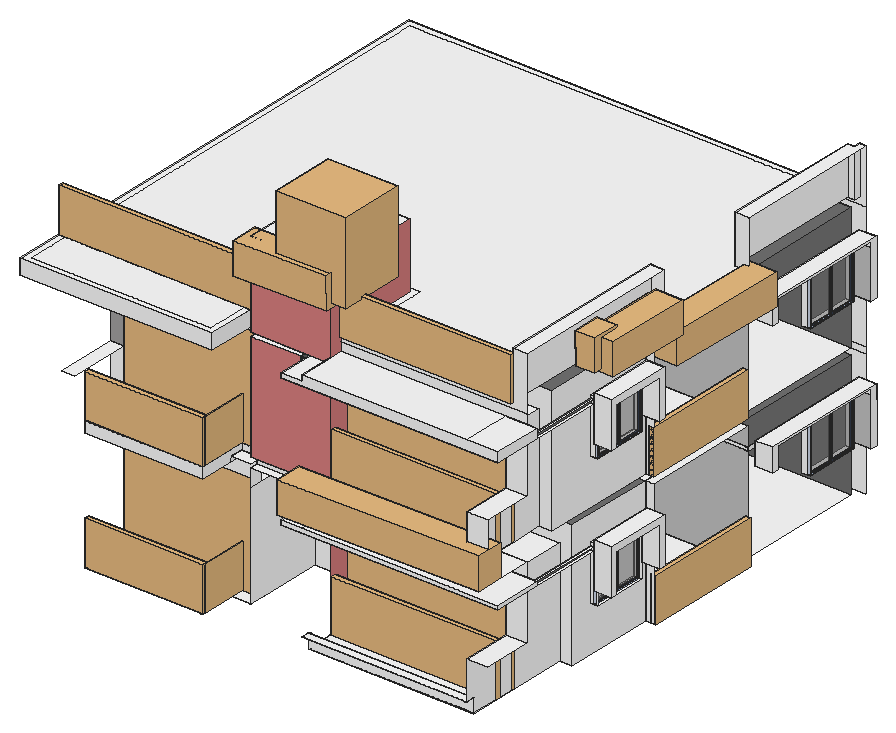
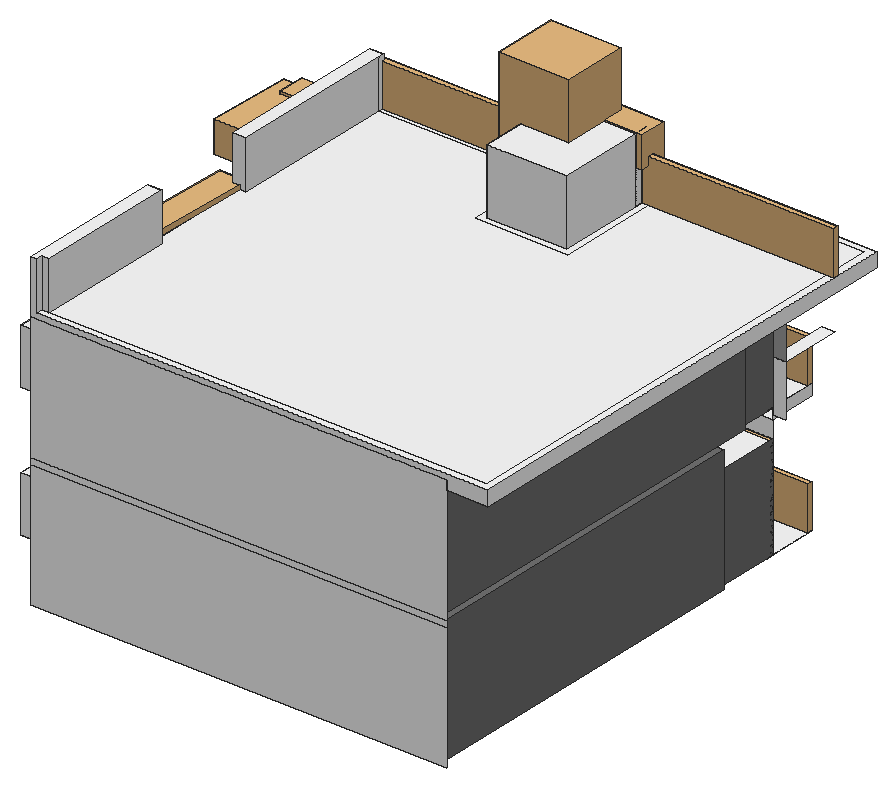
# SketchUp Ruby script. Lengths in inches.
U = 1.inch
M = Sketchup.active_model
def pt(a) = Geom::Point3d.new(a.map { |v| v * U })
def face(e, loops, mat)
  f = e.add_face(loops[0].map { |a| pt(a) })
  loops[1..].each { |l| e.add_face(l.map { |a| pt(a) }).erase! }
  f.material = f.back_material = mat if mat
  f
end
# faces: each face lists its corners as indices into pts; further lists are holes
def faces(e, pts, list, mat = nil) = list.each { |f| face(e, (f[0].is_a?(Array) ? f : [f]).map { |l| l.map { |i| pts[i] } }, mat) }
# xy, xz, yz: faces in a plane at the given z, y or x. An outline is a flat list of corners, or four numbers for a rectangle; further outlines are holes
def ring(l) = l.size == 4 ? [[l[0], l[1]], [l[2], l[1]], [l[2], l[3]], [l[0], l[3]]] : l.each_slice(2).to_a
def flat(e, list, mat, &to3) = list.each { |f| face(e, (f[0].is_a?(Array) ? f : [f]).map { |l| ring(l).map { |u, v| to3.(u, v) } }, mat) }
def xy(e, z, list, mat = nil) = flat(e, list, mat) { |x, y| [x, y, z] }
def xz(e, y, list, mat = nil) = flat(e, list, mat) { |x, z| [x, y, z] }
def yz(e, x, list, mat = nil) = flat(e, list, mat) { |y, z| [x, y, z] }
def lines(e, pts, list) = list.each { |a, b| e.add_line(pt(pts[a]), pt(pts[b])) }
# prism: a flat outline (further loops are holes) pulled along v
def prism(e, loops, v, mat = nil)
  f = face(e, loops, mat); d = Geom::Vector3d.new(v.map { |x| x * U })
  f.pushpull(f.normal.samedirection?(d) ? d.length : -d.length)
end
def box(e, o, s, mat = nil) = prism(e, [[o, [o[0] + s[0], o[1], o[2]], [o[0] + s[0], o[1] + s[1], o[2]], [o[0], o[1] + s[1], o[2]]]], [0, 0, s[2]], mat)
def at(x, y, z, deg = 0) = Geom::Transformation.translation(pt([x, y, z])) * Geom::Transformation.rotation(ORIGIN, Z_AXIS, deg.degrees)
def axes(o, x, y, z) = Geom::Transformation.new([*x, 0, *y, 0, *z, 0, *pt(o).to_a, 1])
def part(name) = M.definitions.add(name)
# library, detail: a bought-in or finely detailed component or shape, given as its bounding box
def library(name, o, s) = part(name).tap { |d| box(d.entities, o, s) }
def detail(e, o, s) = box(e.add_group.entities, o, s)
def put(e, d, t, mat = nil) = e.add_instance(d, t).tap { |i| i.material = mat if mat }
def group(e, t, mat = nil) = e.add_group.tap { |g| g.transformation = t; g.material = mat if mat }.entities
root = M.entities
M.materials.add("[Color M00]").color = [255, 255, 255]
M.materials.add("[Color M02]").color = [198, 198, 198]
M.materials.add("[Color M05]").color = [114, 114, 114]
M.materials.add("[Color M06]").color = [86, 86, 86]
M.materials.add("[Color_006]").color = [86, 86, 86]
M.materials.add("[Stone Vein Gray]").color = [166, 165, 165]
M.materials.add("[Tile Various Tan]").color = [221, 130, 130]
M.materials.add("[Translucent Glass Blue]").color = [74, 111, 178]
M.materials["[Translucent Glass Blue]"].alpha = 0.26
M.materials.add("[Translucent Glass Gray]").color = [128, 128, 128]
M.materials["[Translucent Glass Gray]"].alpha = 0.5
M.materials.add("[Translucent_Glass_Gray]").color = [167, 187, 214]
M.materials["[Translucent_Glass_Gray]"].alpha = 0.8
c1 = library("Glazed balcony doors",[0,0,0],[135.86,2.83,115.35])
c2 = library("Glass Railing",[0,0,0],[139.5,4.76,42])
c3 = part("glass-railing")
detail(c3.entities,[0,0,0],[1.26,75.59,33.1875])
c4 = part("Group\#3")
xy(c4.entities,0,[[0,0,32.48,1.97]])
xy(c4.entities,0.98,[[0.98,0,31.5,0.98],[0.98,0.98,31.5,1.97]])
xy(c4.entities,8.86,[[0.98,0,31.5,0.98],[0.98,0.98,31.5,1.97]])
xy(c4.entities,9.84,[[0,0,32.48,1.97]])
xz(c4.entities,0,[[[0,0,32.48,9.84],[0.98,0.98,31.5,8.86]]])
xz(c4.entities,0.98,[[0.98,0.98,31.5,8.86]],"[Translucent Glass Gray]")
xz(c4.entities,1.97,[[[0,0,32.48,9.84],[0.98,0.98,31.5,8.86]]])
yz(c4.entities,0,[[0,0,1.97,9.84]])
yz(c4.entities,0.98,[[0,0.98,0.98,8.86],[0.98,0.98,1.97,8.86]])
yz(c4.entities,31.5,[[0,0.98,0.98,8.86],[0.98,0.98,1.97,8.86]])
yz(c4.entities,32.48,[[0,0,1.97,9.84]])
c5 = part("Group\#4")
xy(c5.entities,0,[[0,0,32.48,1.97]])
xy(c5.entities,0.98,[[0.98,0,31.5,0.98],[0.98,0.98,31.5,1.97]])
xy(c5.entities,71.85,[[0.98,0,31.5,0.98],[0.98,0.98,31.5,1.97]])
xy(c5.entities,72.83,[[0,0,32.48,1.97]])
xz(c5.entities,0,[[[0,0,32.48,72.83],[0.98,0.98,31.5,71.85]]])
xz(c5.entities,0.98,[[0.98,0.98,31.5,71.85]],"[Translucent Glass Gray]")
xz(c5.entities,1.97,[[[0,0,32.48,72.83],[0.98,0.98,31.5,71.85]]])
yz(c5.entities,0,[[0,0,1.97,72.83]])
yz(c5.entities,0.98,[[0,0.98,0.98,71.85],[0.98,0.98,1.97,71.85]])
yz(c5.entities,31.5,[[0,0.98,0.98,71.85],[0.98,0.98,1.97,71.85]])
yz(c5.entities,32.48,[[0,0,1.97,72.83]])
c6 = part("Fixed transom window")
xy(c6.entities,0,[[0,0,70.86,3.9375]])
xy(c6.entities,1.97,[[1.97,0,34.45,0.98],[36.42,0,68.9,3.9375],[1.97,2.95,34.45,3.9375]])
xy(c6.entities,86.61,[[1.97,0,34.45,3.9375],[34.45,0,36.42,3.9375],[36.42,0,68.9,3.9375]])
xy(c6.entities,88.58,[[0,0,70.86,3.9375]])
xz(c6.entities,0,[[[0,0,70.86,88.58],[1.97,1.97,34.45,86.61],[36.42,1.97,68.9,86.61]]])
xz(c6.entities,3.9375,[[[0,0,70.86,88.58],[1.97,1.97,34.45,86.61],[36.42,1.97,68.9,86.61]]])
yz(c6.entities,0,[[0,0,3.9375,88.58]])
yz(c6.entities,1.97,[[0,1.97,3.9375,74.8],[0,76.77,3.9375,86.61]])
yz(c6.entities,34.45,[[0,1.97,3.9375,86.61]])
yz(c6.entities,36.42,[[0,1.97,3.9375,86.61]])
yz(c6.entities,68.9,[[0,1.97,3.9375,86.61]])
yz(c6.entities,70.86,[[0,0,3.9375,88.58]])
g1 = group(c6.entities,at(1.97,0,74.8))
box(g1,[0,0,0],[66.93,3.9375,1.97])
put(c6.entities,c4,at(1.97,0.98,76.77),"[Translucent Glass Blue]")
put(c6.entities,c4,at(36.42,0.98,76.77),"[Translucent Glass Blue]")
put(c6.entities,c5,at(1.97,0.98,1.97),"[Translucent Glass Blue]")
put(c6.entities,c5,at(36.42,0.98,1.97),"[Translucent Glass Blue]")
c7 = part("FIXED+GLASS+WINDOW+WITH+TRANSOM")
put(c7.entities,c6,at(0,0,0),"[Translucent Glass Blue]")
c8 = part("BIC_Bike Shop - Window - Small")
xy(c8.entities,-8,[[[0,0,36,36],[2,2,34,34]]],"[Color_006]")
xy(c8.entities,-4,[[2,2,34,34]],"[Translucent_Glass_Gray]")
xy(c8.entities,0,[[[0,0,36,36],[2,2,34,34]]],"[Color_006]")
xz(c8.entities,0,[[0,-8,36,0]],"[Color_006]")
xz(c8.entities,2,[[2,-8,34,-4],[2,-4,34,0]],"[Color_006]")
xz(c8.entities,34,[[2,-8,34,-4],[2,-4,34,0]],"[Color_006]")
xz(c8.entities,36,[[0,-8,36,0]],"[Color_006]")
yz(c8.entities,0,[[0,-8,36,0]],"[Color_006]")
yz(c8.entities,2,[[2,-8,34,-4],[2,-4,34,0]],"[Color_006]")
yz(c8.entities,34,[[2,-8,34,-4],[2,-4,34,0]],"[Color_006]")
yz(c8.entities,36,[[0,-8,36,0]],"[Color_006]")
c9 = library("Living wall panel",[-0.54,-4.26,-5.13],[55.52,26.12,125.59])
c10 = library("Flora+17",[-57.52,158.6,-38.64],[66.99,62.88,77.28])
xy(root,635.5625,[[73.74,83.25,73.74,137.58,204.98,137.58,204.98,117.625,186.35,117.625,186.35,83.25],[281.18,91.3,439.11,137.58],[73.74,137.58,204.98,137.58,204.98,194.2,281.18,194.2,281.18,137.58,439.11,137.58,439.11,194.2,450.92,194.2,450.92,281.78,343.48,281.78,343.48,394.46,450.92,394.46,450.92,527.42,69.2,527.42,69.2,194.2,73.74,194.2],[343.48,281.78,450.92,290.48],[450.92,281.78,458.625,394.46],
  [343.48,290.48,352.1875,394.46],[352.1875,290.48,450.92,394.46]],"[Color M00]")
xy(root,635.8125,[[73.74,83.25,186.35,83.25,186.35,117.625,204.98,117.625,204.98,137.58,73.74,137.58],[281.18,91.3,439.11,137.58]],"[Color M00]")
xy(root,649,[[281.18,83.25,439.11,91.3]],"[Color M00]")
xy(root,649.25,[[281.18,83.25,439.11,91.3]],"[Color M00]")
xy(root,679.98,[[450.92,215.57,458.625,267.63],[450.92,468.92,458.625,520.98]],"[Color M00]")
xy(root,685.84,[[439.11,83.25,458.625,129.875]],"[Color M00]")
xy(root,686.24,[[458.625,520.98,475.1875,526.98]],"[Color M00]")
xy(root,694.95,[[458.625,210.07,475.5625,215.57],[458.625,267.63,475.5625,273.63]],"[Color M00]")
xy(root,717.36,[[458.625,402.98,475.1875,408.98]],"[Color M00]")
xy(root,718.41,[[252.64,117.625,281.18,122.0625]],"[Tile Various Tan]")
xy(root,729.27,[[456.375,130.82,458.625,210.07]],"[Color M00]")
xy(root,732.05,[[450.92,215.57,458.625,267.63],[458.625,215.57,475.5625,267.63],[450.92,468.92,458.625,520.98]],"[Color M00]")
xy(root,733.27,[[456.375,130.82,458.625,210.07]],"[Color M00]")
xy(root,734.19,[[381.625,394.46,385.6875,394.83],[385.6875,394.46,401.8125,394.83],[401.8125,394.46,458.625,394.83]],"[Color M00]")
xy(root,734.48,[[73.74,129.875,204.98,194.2]],"[Color M00]")
xy(root,736.125,[[281.18,129.875,439.11,194.2]],"[Color M00]")
xy(root,737.48,[[381.625,394.46,385.6875,394.83],[385.6875,394.46,401.8125,394.83],[401.8125,394.46,458.625,394.83],[458.625,394.46,459,400.46]],"[Color M00]")
xy(root,737.49,[[458.625,408.98,475.1875,520.98]],"[Color M02]")
xy(root,738.39,[[261.54,83.25,261.54,122.0625,281.18,122.0625,281.18,129.875,468.99,129.875,468.99,83.25]],"[Color M00]")
xy(root,738.39,[[252.64,117.625,261.54,122.0625]],"[Tile Various Tan]")
xy(root,738.64,[[458.625,210.07,475.5625,273.63]],"[Color M00]")
xy(root,739.3,[[458.625,402.98,475.1875,526.98]],"[Color M00]")
xy(root,742.08,[[261.54,83.25,281.18,117.625],[281.18,83.25,468.99,129.875]],"[Color M00]")
xy(root,750.9375,[[[73.74,83.25,186.35,129.875],[129.49,93.91,131.04,94.12,132.49,94.72,133.73,95.67,134.68,96.91,135.28,98.36,135.49,99.91,135.28,101.46,134.68,102.91,133.73,104.15,132.49,105.11,131.04,105.71,129.49,105.91,127.93,105.71,126.49,105.11,125.24,104.15,124.29,102.91,123.69,101.46,123.49,99.91,123.69,98.36,124.29,96.91,125.24,95.67,126.49,94.72,127.93,94.12]]],"[Color M00]")
xy(root,752.39,[[204.98,117.625,279.24,125.0625]],"[Color M00]")
xy(root,752.8125,[[129.49,93.91,127.93,94.12,126.49,94.72,125.24,95.67,124.29,96.91,123.69,98.36,123.49,99.91,123.69,101.46,124.29,102.91,125.24,104.15,126.49,105.11,127.93,105.71,129.49,105.91,131.04,105.71,132.49,105.11,133.73,104.15,134.68,102.91,135.28,101.46,135.49,99.91,135.28,98.36,134.68,96.91,133.73,95.67,132.49,94.72,131.04,94.12]],"[Color M06]")
xy(root,755.5625,[[281.18,83.25,458.625,129.875],[186.35,117.625,204.98,129.875],[279.24,117.625,281.18,117.625,281.18,129.875,204.98,129.875,204.98,125.0625,279.24,125.0625],[343.48,281.78,450.92,290.48],[450.92,281.78,450.92,290.48,352.1875,290.48,352.1875,394.46,458.625,394.46,458.625,281.78],
  [343.48,290.48,352.1875,394.46]],"[Color M00]")
xy(root,755.5625,[[69.2,194.2,69.2,527.42,450.92,527.42,450.92,394.46,343.48,394.46,343.48,281.78,450.92,281.78,450.92,194.2]],"[Color M05]")
xy(root,761.5625,[[73.74,83.25,73.74,137.58,204.98,137.58,204.98,129.875,186.35,129.875,186.35,83.25],[281.18,91.3,439.11,137.58],[204.98,117.625,281.18,129.875],[204.98,129.875,281.18,169.45],[73.74,137.58,204.98,137.58,204.98,169.45,281.18,169.45,281.18,137.58,439.11,137.58,439.11,169.45,450.92,169.45,450.92,281.78,343.48,281.78,343.48,394.46,450.92,394.46,450.92,527.42,69.2,527.42,69.2,169.45,73.74,169.45],
  [343.48,281.78,352.1875,290.48],[352.1875,281.78,450.92,290.48],[450.92,281.78,458.625,394.46],[343.48,290.48,352.1875,394.46],[352.1875,290.48,450.92,394.46]],"[Color M00]")
xy(root,761.8125,[[73.74,83.25,186.35,83.25,186.35,129.875,204.98,129.875,204.98,137.58,73.74,137.58],[281.18,91.3,439.11,137.58]],"[Color M00]")
xy(root,775,[[281.18,83.25,439.11,91.3]],"[Color M00]")
xy(root,775.25,[[281.18,83.25,439.11,91.3]],"[Color M00]")
xy(root,805.18,[[61.5,71.125,73.74,129.875]],"[Color M00]")
xy(root,805.98,[[450.92,215.57,458.625,267.63],[450.92,468.92,458.625,520.98]],"[Color M00]")
xy(root,811.84,[[439.11,83.25,458.625,129.875]],"[Color M00]")
xy(root,812.24,[[458.625,520.98,475.1875,526.98]],"[Color M00]")
xy(root,820.95,[[458.625,210.07,475.5625,215.57],[458.625,267.63,475.5625,273.63]],"[Color M00]")
xy(root,843.36,[[458.625,402.98,475.1875,408.98]],"[Color M00]")
xy(root,844.41,[[252.64,117.625,281.18,122.0625]],"[Tile Various Tan]")
xy(root,855.27,[[456.375,130.82,458.625,210.07]],"[Color M00]")
xy(root,858.05,[[450.92,215.57,458.625,267.63],[458.625,215.57,475.5625,267.63],[450.92,468.92,458.625,520.98]],"[Color M00]")
xy(root,859.27,[[456.375,130.82,458.625,210.07]],"[Color M00]")
xy(root,860.19,[[381.625,394.46,385.6875,396.71],[385.6875,394.46,401.8125,396.71],[401.8125,394.46,458.625,396.71]],"[Color M00]")
xy(root,860.48,[[73.74,129.875,204.98,169.45]],"[Color M00]")
xy(root,862.125,[[281.18,129.875,439.11,169.45]],"[Color M00]")
xy(root,863.48,[[381.625,394.46,385.6875,396.71],[385.6875,394.46,401.8125,396.71],[401.8125,394.46,458.625,396.71],[458.625,394.46,459,400.46]],"[Color M00]")
xy(root,863.49,[[458.625,408.98,475.1875,520.98]],"[Color M00]")
xy(root,864.39,[[261.54,83.25,261.54,122.0625,281.18,122.0625,281.18,129.875,468.99,129.875,468.99,83.25],[204.98,117.625,252.64,117.625,252.64,122.0625,261.54,122.0625,261.54,137.1875,204.98,137.1875]],"[Color M00]")
xy(root,864.64,[[458.625,210.07,475.5625,273.63]],"[Color M00]")
xy(root,865.3,[[458.625,402.98,475.1875,526.98]],"[Color M00]")
xy(root,868.08,[[261.54,83.25,281.18,117.625],[204.98,117.625,261.54,137.1875]],"[Color M00]")
xy(root,873.0625,[[[22.125,71.125,22.125,535.125,61.5,535.125,61.5,129.875,204.98,129.875,204.98,71.125],[124.6,84.17,126.16,84.38,127.6,84.98,128.85,85.93,129.8,87.17,130.4,88.62,130.6,90.17,130.4,91.73,129.8,93.17,128.85,94.42,127.6,95.37,126.16,95.97,124.6,96.17,123.05,95.97,121.6,95.37,120.36,94.42,119.41,93.17,118.81,91.73,118.6,90.17,118.81,88.62,119.41,87.17,120.36,85.93,121.6,84.98,123.05,84.38]]],"[Color M00]")
xy(root,873.08,[[281.18,83.25,439.24,129.875],[439.24,83.25,468.99,129.875]],"[Color M00]")
xy(root,874.9375,[[124.6,84.17,123.05,84.38,121.6,84.98,120.36,85.93,119.41,87.17,118.81,88.62,118.6,90.17,118.81,91.73,119.41,93.17,120.36,94.42,121.6,95.37,123.05,95.97,124.6,96.17,126.16,95.97,127.6,95.37,128.85,94.42,129.8,93.17,130.4,91.73,130.6,90.17,130.4,88.62,129.8,87.17,128.85,85.93,127.6,84.98,126.16,84.38]],"[Color M06]")
xy(root,881.5625,[[343.48,281.78,352.1875,290.48],[352.1875,281.78,450.92,290.48],[450.92,281.78,450.92,290.48,352.1875,290.48,352.1875,394.46,458.625,394.46,458.625,281.78],[343.48,290.48,352.1875,394.46]],"[Color M00]")
xy(root,881.5625,[[69.2,169.45,69.2,527.42,450.92,527.42,450.92,394.46,343.48,394.46,343.48,281.78,450.92,281.78,450.92,169.45]],"[Color M05]")
xy(root,887.5625,[[22.125,71.125,204.98,71.125,204.98,212.5625,281.18,212.5625,281.18,129.875,445.9,129.875,445.9,135.91,287.21,135.91,287.21,218.6,198.94,218.6,198.94,77.16,28.16,77.16,28.16,529.09,452.59,529.09,452.59,535.125,22.125,535.125],[28.16,77.16,198.94,77.16,198.94,218.6,287.21,218.6,287.21,135.91,445.9,135.91,445.9,293.73,452.59,293.73,452.59,395.21,445.9,395.21,445.9,529.09,28.16,529.09],[452.59,293.73,458.625,395.21]],"[Color M00]")
xy(root,898.34,[[458.625,209.21,475.5625,275.34]],"[Color M00]")
xy(root,921.66,[[458.625,209.21,475.5625,275.34]],"[Color M00]")
xy(root,933.5,[[445.9,129.875,458.625,293.73],[445.9,395.21,458.625,395.21,458.625,535.125,452.59,535.125,452.59,529.09,445.9,529.09]],"[Color M00]")
xy(root,950.125,[[204.98,117.625,281.18,129.875],[204.98,129.875,281.18,212.5625]],"[Color M00]")
xz(root,71.125,[[22.125,873.0625,204.98,887.5625]],"[Color M00]")
xz(root,83.25,[[73.74,635.5625,186.35,635.8125],[281.18,649,439.11,649.25],[261.54,738.39,468.99,742.08],[73.74,750.9375,186.35,761.5625],[281.18,755.5625,458.625,755.5625,458.625,811.84,439.11,811.84,439.11,775,281.18,775],
  [73.74,761.5625,186.35,761.8125],[281.18,775,439.11,775.25],[261.54,864.39,468.99,864.39,468.99,873.08,281.18,873.08,281.18,868.08,261.54,868.08]],"[Color M00]")
xz(root,91.3,[[281.18,635.5625,439.11,635.8125],[281.18,635.8125,439.11,649],[281.18,649,439.11,649.25],[281.18,761.5625,439.11,761.8125],[281.18,761.8125,439.11,775],
  [281.18,775,439.11,775.25]],"[Color M00]")
xz(root,117.625,[[186.35,635.5625,204.98,635.8125],[279.24,742.08,281.18,755.5625]],"[Color M00]")
xz(root,117.625,[[204.98,761.5625,281.18,761.5625,281.18,844.41,252.64,844.41,252.64,864.39,204.98,864.39],[204.98,868.08,281.18,950.125]],"[Tile Various Tan]")
xz(root,122.0625,[[252.64,718.41,281.18,738.39],[252.64,844.41,281.18,864.39]],"[Tile Various Tan]")
xz(root,125.0625,[[204.98,752.39,279.24,755.5625]],"[Color M00]")
xz(root,129.875,[[439.11,685.84,458.625,685.84,458.625,738.39,281.18,738.39,281.18,736.125,439.11,736.125],[73.74,734.48,204.98,734.48,204.98,755.5625,186.35,755.5625,186.35,750.9375,73.74,750.9375],[439.24,738.39,458.625,742.08],[458.625,738.39,468.99,742.08],[281.18,742.08,458.625,755.5625],
  [61.5,755.5625,73.74,805.18],[186.35,755.5625,281.18,761.5625],[186.35,761.5625,204.98,761.8125],[439.11,811.84,458.625,811.84,458.625,864.39,281.18,864.39,281.18,862.125,439.11,862.125],[73.74,860.48,204.98,873.0625],
  [439.24,864.39,458.625,873.08],[458.625,864.39,468.99,873.08],[61.5,873.0625,204.98,881.5625],[281.18,873.08,458.625,881.5625],[281.18,881.5625,458.625,881.5625,458.625,933.5,445.9,933.5,445.9,887.5625,281.18,887.5625]],"[Color M00]")
xz(root,129.875,[[61.5,805.18,73.74,873.0625]],"[Stone Vein Gray]")
xz(root,130.82,[[456.375,729.27,458.625,733.27],[456.375,855.27,458.625,859.27]],"[Color M00]")
xz(root,137.1875,[[204.98,864.39,261.54,868.08]],"[Color M00]")
xz(root,137.58,[[73.74,635.5625,204.98,635.8125],[281.18,635.5625,439.11,635.8125],[73.74,761.5625,204.98,761.8125],[281.18,761.5625,439.11,761.8125]],"[Color M00]")
xz(root,169.45,[[69.2,761.5625,69.2,881.5625,450.92,881.5625,450.92,761.5625,439.11,761.5625,439.11,862.125,281.18,862.125,281.18,761.5625,204.98,761.5625,204.98,860.48,73.74,860.48,73.74,761.5625]],"[Color M00]")
xz(root,194.2,[[69.2,635.5625,69.2,755.5625,450.92,755.5625,450.92,635.5625,439.11,635.5625,439.11,736.125,281.18,736.125,281.18,635.5625,204.98,635.5625,204.98,734.48,73.74,734.48,73.74,635.5625]],"[Color M00]")
xz(root,209.21,[[458.625,898.34,475.5625,921.66]],"[Color M00]")
xz(root,210.07,[[458.625,694.95,475.5625,738.64],[456.375,729.27,458.625,732.11],[456.375,732.11,458.625,733.27],[458.625,820.95,475.5625,864.64],[456.375,855.27,458.625,858.11],
  [456.375,858.11,458.625,859.27]],"[Color M00]")
xz(root,212.5625,[[204.98,887.5625,281.18,950.125]],"[Color M00]")
xz(root,215.57,[[450.92,679.98,458.625,732.05],[458.625,694.95,475.5625,732.05],[450.92,805.98,458.625,858.05],[458.625,820.95,475.5625,858.05]],"[Color M00]")
xz(root,267.63,[[450.92,679.98,458.625,732.05],[458.625,694.95,475.5625,732.05],[450.92,805.98,458.625,858.05],[458.625,820.95,475.5625,858.05]],"[Color M00]")
xz(root,273.63,[[458.625,694.95,475.5625,738.64],[458.625,820.95,475.5625,864.64]],"[Color M00]")
xz(root,275.34,[[458.625,898.34,475.5625,921.66]],"[Color M00]")
xz(root,281.78,[[343.48,635.5625,450.92,755.5625],[450.92,635.5625,458.625,755.5625],[343.48,761.5625,352.1875,881.5625],[352.1875,761.5625,450.92,881.5625],[450.92,761.5625,458.625,881.5625]],"[Color M00]")
xz(root,290.48,[[343.48,635.5625,352.1875,755.5625],[352.1875,635.5625,450.92,755.5625],[343.48,761.5625,352.1875,881.5625],[352.1875,761.5625,450.92,881.5625]],"[Color M00]")
xz(root,293.73,[[445.9,887.5625,458.625,933.5]],"[Color M00]")
xz(root,394.46,[[343.48,635.5625,352.1875,755.5625],[343.48,761.5625,352.1875,881.5625]],"[Color M00]")
xz(root,394.46,[[352.1875,635.5625,458.625,635.5625,458.625,734.19,381.625,734.19,381.625,737.48,458.625,737.48,458.625,755.5625,352.1875,755.5625],[352.1875,761.5625,458.625,761.5625,458.625,860.19,381.625,860.19,381.625,863.48,458.625,863.48,458.625,881.5625,352.1875,881.5625]],"[Color M02]")
xz(root,394.83,[[381.625,734.19,458.625,737.48]],"[Color M00]")
xz(root,395.21,[[445.9,887.5625,458.625,933.5]],"[Color M00]")
xz(root,396.71,[[381.625,860.19,458.625,863.48]],"[Color M00]")
xz(root,400.46,[[458.625,734.11,459,737.48],[458.625,860.11,459,863.48]],"[Color M00]")
xz(root,402.98,[[458.625,717.36,475.1875,739.3],[458.625,843.36,475.1875,865.3]],"[Color M00]")
xz(root,408.98,[[458.625,717.36,475.1875,731.49],[458.625,731.49,475.1875,737.49],[458.625,843.36,475.1875,857.49],[458.625,857.49,475.1875,863.49]],"[Color M00]")
xz(root,468.92,[[450.92,679.98,458.625,732.05],[450.92,805.98,458.625,858.05]],"[Color M00]")
xz(root,520.98,[[450.92,679.98,458.625,732.05],[458.625,732.05,475.1875,737.49],[450.92,805.98,458.625,858.05],[458.625,858.05,475.1875,863.49]],"[Color M00]")
xz(root,520.98,[[458.625,686.24,475.1875,732.05],[458.625,812.24,475.1875,858.05]],"[Color M02]")
xz(root,526.98,[[458.625,686.24,475.1875,739.3],[458.625,812.24,475.1875,865.3]],"[Color M00]")
xz(root,527.42,[[69.2,635.5625,450.92,755.5625],[69.2,761.5625,450.92,881.5625]],"[Color M05]")
xz(root,529.09,[[445.9,887.5625,452.59,933.5]],"[Color M00]")
xz(root,535.125,[[61.5,635.5625,458.625,755.5625],[61.5,755.5625,458.625,761.5625],[61.5,761.5625,458.625,881.5625],[22.125,873.0625,22.125,887.5625,452.59,887.5625,452.59,933.5,458.625,933.5,458.625,881.5625,61.5,881.5625,61.5,873.0625]],"[Color M00]")
yz(root,22.125,[[71.125,873.0625,535.125,887.5625]],"[Color M00]")
yz(root,61.5,[[129.875,873.0625,535.125,881.5625]],"[Color M00]")
yz(root,69.2,[[194.2,635.5625,527.42,755.5625],[169.45,761.5625,527.42,881.5625]],"[Color M05]")
yz(root,73.74,[[83.25,635.5625,129.875,635.8125],[129.875,635.5625,137.58,635.8125],[83.25,750.9375,129.875,761.5625],[83.25,761.5625,129.875,761.8125],[129.875,761.5625,137.58,761.8125]],"[Color M00]")
yz(root,73.74,[[137.58,635.5625,194.2,635.5625,194.2,734.48,129.875,734.48,129.875,635.8125,137.58,635.8125],[137.58,761.5625,169.45,761.5625,169.45,860.48,129.875,860.48,129.875,761.8125,137.58,761.8125]],"[Color M05]")
yz(root,186.35,[[83.25,635.5625,117.625,635.8125],[83.25,750.9375,117.625,750.9375,117.625,755.5625,129.875,755.5625,129.875,761.5625,83.25,761.5625],[117.625,750.9375,129.875,755.5625],[83.25,761.5625,129.875,761.8125]],"[Color M00]")
yz(root,204.98,[[117.625,635.5625,137.58,635.8125],[137.58,635.5625,137.58,635.8125,117.625,635.8125,117.625,734.48,194.2,734.48,194.2,635.5625],[117.625,734.48,117.625,752.39,125.0625,752.39,125.0625,755.5625,129.875,755.5625,129.875,734.48],[117.625,761.5625,117.625,860.48,169.45,860.48,169.45,761.5625,137.58,761.5625,137.58,761.8125,129.875,761.8125,129.875,761.5625],[129.875,761.5625,137.58,761.8125],
  [117.625,860.48,129.875,864.39],[129.875,864.39,137.1875,868.08],[117.625,868.08,129.875,873.0625],[71.125,873.0625,117.625,887.5625],[117.625,873.0625,129.875,887.5625],
  [117.625,887.5625,129.875,950.125],[129.875,887.5625,212.5625,950.125]],"[Color M00]")
yz(root,252.64,[[117.625,718.41,122.0625,738.39],[117.625,844.41,122.0625,864.39]],"[Tile Various Tan]")
yz(root,261.54,[[83.25,738.39,117.625,742.08],[83.25,864.39,137.1875,868.08]],"[Color M00]")
yz(root,279.24,[[117.625,752.39,125.0625,755.5625]],"[Color M00]")
yz(root,281.18,[[91.3,635.5625,117.625,635.8125],[117.625,635.5625,137.58,635.8125],[83.25,649,91.3,649.25],[122.0625,736.125,129.875,738.39],[117.625,742.08,129.875,755.5625],
  [83.25,755.5625,83.25,775,91.3,775,91.3,761.5625,129.875,761.5625,129.875,755.5625],[91.3,761.5625,117.625,761.8125],[117.625,761.5625,129.875,761.8125],[129.875,761.5625,137.58,761.8125],[83.25,775,91.3,775.25],
  [83.25,868.08,117.625,873.08]],"[Color M00]")
yz(root,281.18,[[137.58,635.5625,194.2,635.5625,194.2,736.125,122.0625,736.125,122.0625,718.41,117.625,718.41,117.625,635.8125,137.58,635.8125],[137.58,761.5625,169.45,761.5625,169.45,862.125,122.0625,862.125,122.0625,844.41,117.625,844.41,117.625,761.8125,137.58,761.8125],[122.0625,862.125,129.875,864.39],[117.625,873.08,129.875,873.08,129.875,887.5625,212.5625,887.5625,212.5625,950.125,117.625,950.125]],"[Tile Various Tan]")
yz(root,343.48,[[281.78,635.5625,290.48,755.5625],[290.48,635.5625,394.46,755.5625],[281.78,761.5625,290.48,881.5625],[290.48,761.5625,394.46,881.5625]],"[Color M00]")
yz(root,352.1875,[[290.48,635.5625,394.46,755.5625],[281.78,761.5625,290.48,881.5625],[290.48,761.5625,394.46,881.5625]],"[Color M00]")
yz(root,381.625,[[394.46,734.19,394.83,737.48],[394.46,860.19,396.71,863.48]],"[Color M00]")
yz(root,439.11,[[137.58,635.5625,137.58,635.8125,91.3,635.8125,91.3,649.25,83.25,649.25,83.25,685.84,129.875,685.84,129.875,736.125,194.2,736.125,194.2,635.5625],[91.3,635.5625,137.58,635.8125],[83.25,649,91.3,649.25],[137.58,761.5625,137.58,761.8125,91.3,761.8125,91.3,775.25,83.25,775.25,83.25,811.84,129.875,811.84,129.875,862.125,169.45,862.125,169.45,761.5625],[91.3,761.5625,137.58,761.8125],
  [83.25,775,91.3,775.25]],"[Color M00]")
yz(root,445.9,[[129.875,887.5625,135.91,933.5],[135.91,887.5625,293.73,933.5],[395.21,887.5625,529.09,933.5]],"[Color M00]")
yz(root,450.92,[[[194.2,635.5625,281.78,755.5625],[215.57,679.98,267.63,732.05]],[281.78,635.5625,290.48,755.5625],[[169.45,761.5625,281.78,881.5625],[215.57,805.98,267.63,858.05]],[281.78,761.5625,290.48,881.5625]],"[Color M00]")
yz(root,452.59,[[529.09,887.5625,535.125,933.5]],"[Color M00]")
yz(root,456.375,[[130.82,729.27,210.07,733.27],[130.82,855.27,210.07,859.27]],"[Color M05]")
yz(root,458.625,[[520.98,686.24,520.98,737.49,408.98,737.49,408.98,717.36,402.98,717.36,402.98,739.3,526.98,739.3,526.98,686.24],[210.07,694.95,210.07,738.64,273.63,738.64,273.63,694.95,267.63,694.95,267.63,732.05,215.57,732.05,215.57,694.95],[394.46,734.19,394.83,737.48],[520.98,812.24,520.98,863.49,408.98,863.49,408.98,843.36,402.98,843.36,402.98,865.3,526.98,865.3,526.98,812.24],[210.07,820.95,210.07,864.64,273.63,864.64,273.63,820.95,267.63,820.95,267.63,858.05,215.57,858.05,215.57,820.95],
  [394.46,860.19,396.71,863.48]],"[Color M00]")
yz(root,459,[[400.46,734.11,400.46,737.48,394.46,737.48,394.46,734.19],[400.46,860.11,400.46,863.48,394.46,863.48,394.46,860.19]],"[Color M00]")
yz(root,468.99,[[83.25,738.39,129.875,742.08],[83.25,864.39,129.875,873.08]],"[Color M00]")
yz(root,475.1875,[[520.98,686.24,526.98,686.24,526.98,739.3,402.98,739.3,402.98,717.36,408.98,717.36,408.98,737.49,520.98,737.49],[520.98,812.24,526.98,812.24,526.98,865.3,402.98,865.3,402.98,843.36,408.98,843.36,408.98,863.49,520.98,863.49]],"[Color M00]")
yz(root,475.5625,[[210.07,694.95,215.57,694.95,215.57,732.05,267.63,732.05,267.63,694.95,273.63,694.95,273.63,738.64,210.07,738.64],[210.07,820.95,215.57,820.95,215.57,858.05,267.63,858.05,267.63,820.95,273.63,820.95,273.63,864.64,210.07,864.64],[209.21,898.34,275.34,921.66]],"[Color M00]")
p = [[459,400.46,734.11],[459,394.46,734.19],[458.625,394.46,734.19],[458.625,400.46,734.11],[129.49,93.91,750.9375],[127.93,94.12,750.9375],
  [127.93,94.12,752.8125],[129.49,93.91,752.8125],[131.04,94.12,750.9375],[131.04,94.12,752.8125],[126.49,94.72,750.9375],[126.49,94.72,752.8125],
  [132.49,94.72,750.9375],[132.49,94.72,752.8125],[125.24,95.67,750.9375],[125.24,95.67,752.8125],[133.73,95.67,750.9375],[133.73,95.67,752.8125],
  [124.29,96.91,750.9375],[124.29,96.91,752.8125],[134.68,96.91,750.9375],[134.68,96.91,752.8125],[123.69,98.36,750.9375],[123.69,98.36,752.8125],
  [135.28,98.36,750.9375],[135.28,98.36,752.8125],[123.49,99.91,750.9375],[123.49,99.91,752.8125],[135.49,99.91,750.9375],[135.49,99.91,752.8125],
  [123.69,101.46,750.9375],[123.69,101.46,752.8125],[135.28,101.46,750.9375],[135.28,101.46,752.8125],[124.29,102.91,750.9375],[124.29,102.91,752.8125],
  [134.68,102.91,750.9375],[134.68,102.91,752.8125],[125.24,104.15,750.9375],[125.24,104.15,752.8125],[133.73,104.15,750.9375],[133.73,104.15,752.8125],
  [126.49,105.11,750.9375],[126.49,105.11,752.8125],[132.49,105.11,750.9375],[132.49,105.11,752.8125],[127.93,105.71,750.9375],[127.93,105.71,752.8125],
  [131.04,105.71,750.9375],[131.04,105.71,752.8125],[129.49,105.91,750.9375],[129.49,105.91,752.8125],[459,400.46,860.11],[459,394.46,860.19],
  [458.625,394.46,860.19],[458.625,400.46,860.11],[124.6,84.17,873.0625],[123.05,84.38,873.0625],[123.05,84.38,874.9375],[124.6,84.17,874.9375],
  [126.16,84.38,873.0625],[126.16,84.38,874.9375],[121.6,84.98,873.0625],[121.6,84.98,874.9375],[127.6,84.98,873.0625],[127.6,84.98,874.9375],
  [120.36,85.93,873.0625],[120.36,85.93,874.9375],[128.85,85.93,873.0625],[128.85,85.93,874.9375],[119.41,87.17,873.0625],[119.41,87.17,874.9375],
  [129.8,87.17,873.0625],[129.8,87.17,874.9375],[118.81,88.62,873.0625],[118.81,88.62,874.9375],[130.4,88.62,873.0625],[130.4,88.62,874.9375],
  [118.6,90.17,873.0625],[118.6,90.17,874.9375],[130.6,90.17,873.0625],[130.6,90.17,874.9375],[118.81,91.73,873.0625],[118.81,91.73,874.9375],
  [130.4,91.73,873.0625],[130.4,91.73,874.9375],[119.41,93.17,873.0625],[119.41,93.17,874.9375],[129.8,93.17,873.0625],[129.8,93.17,874.9375],
  [120.36,94.42,873.0625],[120.36,94.42,874.9375],[128.85,94.42,873.0625],[128.85,94.42,874.9375],[121.6,95.37,873.0625],[121.6,95.37,874.9375],
  [127.6,95.37,873.0625],[127.6,95.37,874.9375],[123.05,95.97,873.0625],[123.05,95.97,874.9375],[126.16,95.97,873.0625],[126.16,95.97,874.9375],
  [124.6,96.17,873.0625],[124.6,96.17,874.9375],[204.98,129.875,881.5625],[281.18,129.875,881.5625]]
faces(root,p,[[0,1,2,3],[52,53,54,55]],"[Color M00]")
faces(root,p,[[4,5,6,7],[8,4,7,9],[5,10,11,6],[12,8,9,13],[10,14,15,11],[16,12,13,17],[14,18,19,15],[20,16,17,21],
  [18,22,23,19],[24,20,21,25],[22,26,27,23],[28,24,25,29],[26,30,31,27],[32,28,29,33],[30,34,35,31],[36,32,33,37],
  [34,38,39,35],[40,36,37,41],[38,42,43,39],[44,40,41,45],[42,46,47,43],[48,44,45,49],[46,50,51,47],[50,48,49,51],
  [56,57,58,59],[60,56,59,61],[57,62,63,58],[64,60,61,65],[62,66,67,63],[68,64,65,69],[66,70,71,67],[72,68,69,73],
  [70,74,75,71],[76,72,73,77],[74,78,79,75],[80,76,77,81],[78,82,83,79],[84,80,81,85],[82,86,87,83],[88,84,85,89],
  [86,90,91,87],[92,88,89,93],[90,94,95,91],[96,92,93,97],[94,98,99,95],[100,96,97,101],[98,102,103,99],[102,100,101,103]],"[Color M06]")
lines(root,p,[[104,105]])
put(root,c1,axes([73.74,129.875,635.3125],[0.96594,0,0],[0,0.86,0],[0,0,0.86]),"[Color M00]")
put(root,c2,axes([461.04,281.78,635.53],[0,0.80723,0],[-1,0,0],[0,0,1]),"[Color M00]")
put(root,c2,axes([281.18,117.625,635.5625],[1.13217,0,0],[0,1,0],[0,0,1.19717]),"[Color M00]")
put(root,c1,axes([281.18,136.9375,635.8125],[1.16249,0,0],[0,0.86,0],[0,0,0.86]),"[Color M00]")
put(root,c2,axes([73.74,83.25,635.8125],[0.80723,0,0],[0,1,0],[0,0,1]),"[Color M00]")
put(root,c3,axes([186.35,85.95,636.03],[1,0,0],[0,1,0],[0,0,1.24195]),"[Color M00]")
put(root,c7,axes([457.01,215.57,679.98],[0,0.73468,0],[-0.59,0,0],[0,0,0.59]),"[Color M00]")
put(root,c7,axes([458.625,468.92,679.98],[0,0.73244,0],[-0.59,0,0],[0,0,0.57689]),"[Color M00]")
put(root,c8,axes([252.64,117.625,718.41],[0.79273,0,0],[0,0,0.56],[0,-0.56,0]))
put(root,c9,axes([275.83,74.53,784.6875],[0.0058,0,-0.53997],[0,1,0],[1.53606,0,0.0165]),"[Color M00]")
put(root,c2,axes([73.74,83.25,761.5625],[0.80723,0,0],[0,1,0],[0,0,1]),"[Color M00]")
put(root,c2,axes([281.18,117.625,761.5625],[1.13217,0,0],[0,1,0],[0,0,1.19717]),"[Color M00]")
put(root,c2,axes([458.625,281.78,761.5625],[0,0.80723,0],[-1,0,0],[0,0,1]),"[Color M00]")
put(root,c1,axes([73.74,129.875,761.8125],[0.96594,0,0],[0,0.86,0],[0,0,0.86]),"[Color M00]")
put(root,c1,axes([281.18,136.9375,761.8125],[1.16249,0,0],[0,0.86,0],[0,0,0.86]),"[Color M00]")
put(root,c3,axes([186.35,85.95,762.28],[1,0,0],[0,1,0],[0,0,1.24195]),"[Color M00]")
put(root,c7,axes([458.625,215.57,805.98],[0,0.73468,0],[-0.59,0,0],[0,0,0.59]),"[Color M00]")
put(root,c7,axes([458.625,468.92,805.98],[0,0.73244,0],[-0.59,0,0],[0,0,0.57689]),"[Color M00]")
put(root,c8,axes([252.64,117.625,844.41],[0.79273,0,0],[0,0,0.56],[0,-0.56,0]))
put(root,c9,axes([473.8,290.21,890.71],[0.00013,0.0058,-0.53997],[-0.99974,0.02269,0],[0.0209,0.9209,0.0099]),"[Color M00]")
put(root,c2,axes([281.18,127.13,886.875],[1.18084,0,0],[0,1,0],[0,0,1]),"[Color M00]")
put(root,c2,axes([22.125,117.625,887.5625],[1.31077,0,0],[0,1,0],[0,0,1]),"[Color M00]")
put(root,c9,axes([485.07,198.33,925.27],[0.00013,0.0058,-0.53997],[-0.99974,0.02269,0],[0.01463,0.64463,0.00693]),"[Color M00]")
put(root,c9,axes([459.39,192.32,927.375],[0.0058,0,-0.53997],[0,1,0],[0.14903,0,0.0016]),"[Color M00]")
put(root,c9,axes([202.76,108.02,950.28],[0.0058,0,-0.53997],[0,1,0],[0.70966,0,0.00762]),"[Color M00]")
put(root,c10,at(293.22,-49.68,965.02))
